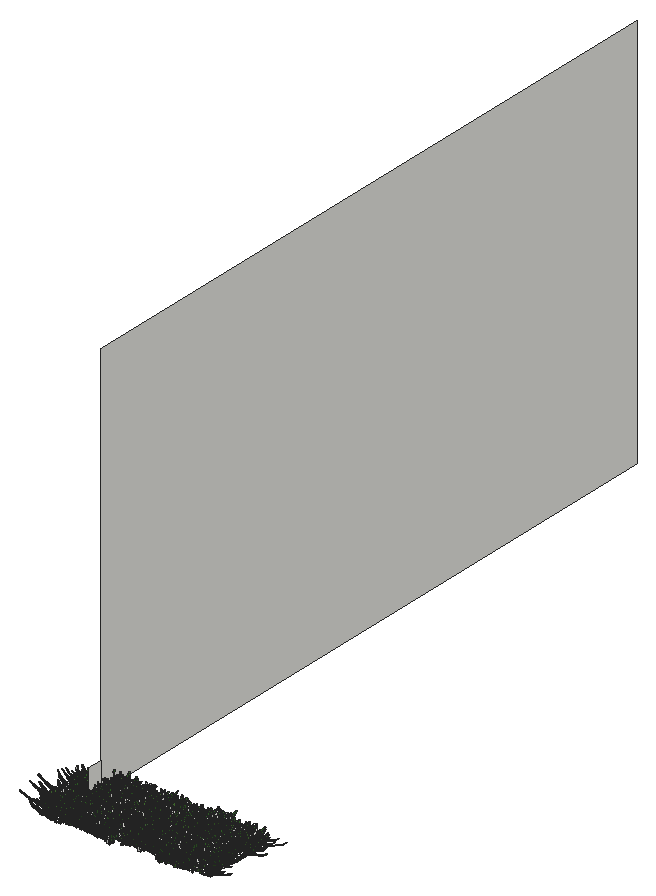
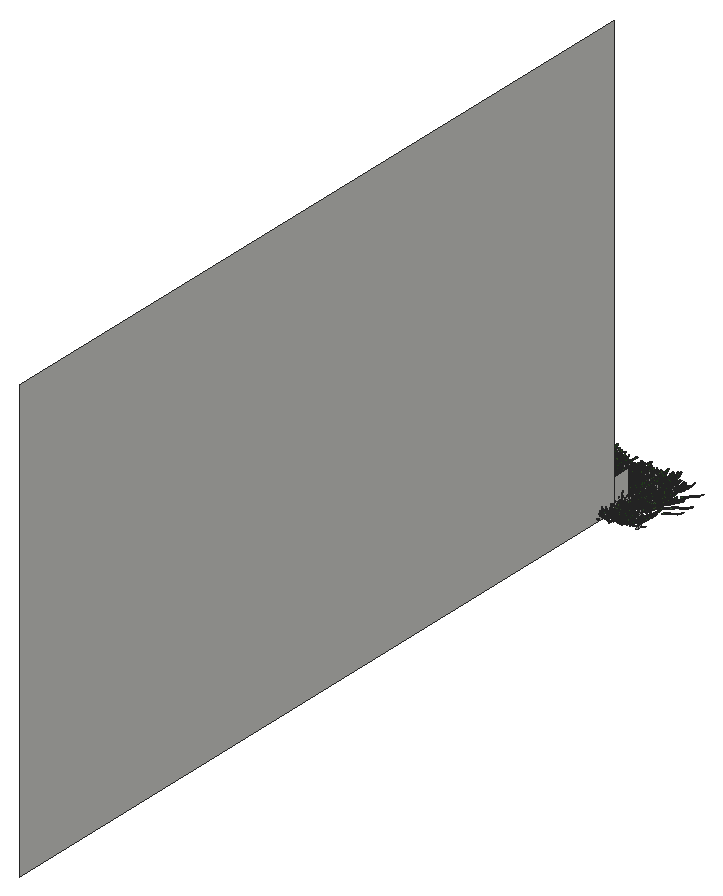
# SketchUp Ruby script. Lengths in inches.
U = 1.inch
M = Sketchup.active_model
def pt(a) = Geom::Point3d.new(a.map { |v| v * U })
def face(e, loops, mat)
  f = e.add_face(loops[0].map { |a| pt(a) })
  loops[1..].each { |l| e.add_face(l.map { |a| pt(a) }).erase! }
  f.material = f.back_material = mat if mat
  f
end
# faces: each face lists its corners as indices into pts; further lists are holes
def faces(e, pts, list, mat = nil) = list.each { |f| face(e, (f[0].is_a?(Array) ? f : [f]).map { |l| l.map { |i| pts[i] } }, mat) }
# xy, xz, yz: faces in a plane at the given z, y or x. An outline is a flat list of corners, or four numbers for a rectangle; further outlines are holes
def ring(l) = l.size == 4 ? [[l[0], l[1]], [l[2], l[1]], [l[2], l[3]], [l[0], l[3]]] : l.each_slice(2).to_a
def flat(e, list, mat, &to3) = list.each { |f| face(e, (f[0].is_a?(Array) ? f : [f]).map { |l| ring(l).map { |u, v| to3.(u, v) } }, mat) }
def xy(e, z, list, mat = nil) = flat(e, list, mat) { |x, y| [x, y, z] }
def xz(e, y, list, mat = nil) = flat(e, list, mat) { |x, z| [x, y, z] }
def yz(e, x, list, mat = nil) = flat(e, list, mat) { |y, z| [x, y, z] }
def lines(e, pts, list) = list.each { |a, b| e.add_line(pt(pts[a]), pt(pts[b])) }
# prism: a flat outline (further loops are holes) pulled along v
def prism(e, loops, v, mat = nil)
  f = face(e, loops, mat); d = Geom::Vector3d.new(v.map { |x| x * U })
  f.pushpull(f.normal.samedirection?(d) ? d.length : -d.length)
end
def box(e, o, s, mat = nil) = prism(e, [[o, [o[0] + s[0], o[1], o[2]], [o[0] + s[0], o[1] + s[1], o[2]], [o[0], o[1] + s[1], o[2]]]], [0, 0, s[2]], mat)
def at(x, y, z, deg = 0) = Geom::Transformation.translation(pt([x, y, z])) * Geom::Transformation.rotation(ORIGIN, Z_AXIS, deg.degrees)
def axes(o, x, y, z) = Geom::Transformation.new([*x, 0, *y, 0, *z, 0, *pt(o).to_a, 1])
def part(name) = M.definitions.add(name)
# library, detail: a bought-in or finely detailed component or shape, given as its bounding box
def library(name, o, s) = part(name).tap { |d| box(d.entities, o, s) }
def detail(e, o, s) = box(e.add_group.entities, o, s)
def put(e, d, t, mat = nil) = e.add_instance(d, t).tap { |i| i.material = mat if mat }
def group(e, t, mat = nil) = e.add_group.tap { |g| g.transformation = t; g.material = mat if mat }.entities
root = M.entities
M.materials.add("Material82").color = [68, 110, 58]
M.materials.add("Material83").color = [48, 90, 38]
M.materials.add("Material84").color = [68, 110, 48]
M.materials.add("Material85").color = [48, 90, 48]
M.materials.add("Material86").color = [58, 110, 58]
M.materials.add("Material87").color = [58, 90, 38]
M.materials.add("Material88").color = [68, 100, 58]
M.materials.add("Material89").color = [48, 100, 38]
c1 = part("grass00")
p = [[-0.6875,0.15,0],[-0.56,0.08,5.52],[-0.04,0.03,2.76],[0.48,-0.02,0],[0.35,-0.02,5.52],[-0.1,-0.14,5.52],
  [-0.12,0.65,8.37],[-0.42,0.65,8.37]]
faces(c1.entities,p,[[0,1,2,3],[3,2,4],[1,5,2],[5,4,2],[1,6,5],[4,5,6],[7,6,1]])
c2 = part("Group16\#1")
put(c2.entities,c1,axes([1.44,-0.61,-0.01],[0.05352,0.12609,0],[-0.10704,0.04543,0.07239],[0.06664,-0.02828,0.11628]),"Material85")
put(c2.entities,c1,axes([0.76,-0.15,-0.01],[0.04676,0.24062,0],[-0.23162,0.04501,0.06642],[0.0652,-0.01267,0.23595]),"Material82")
put(c2.entities,c1,axes([0.79,0.01,-0.01],[-0.00606,0.34651,0],[-0.34381,-0.00602,0.0432],[0.04319,0.00076,0.34386]))
put(c2.entities,c1,axes([1,0.23,-0.01],[-0.07192,0.31144,0],[-0.28722,-0.06632,0.1236],[0.12043,0.02781,0.29478]),"Material84")
put(c2.entities,c1,axes([1.66,0.77,-0.01],[-0.13828,0.29651,0],[-0.21551,-0.1005,0.22471],[0.20365,0.09498,0.23779]),"Material89")
put(c2.entities,c1,axes([0.6875,0.52,-0.01],[-0.18126,0.24051,0],[-0.22746,-0.17142,0.09788],[0.07817,0.05891,0.28481]),"Material84")
put(c2.entities,c1,axes([0.68,0.78,-0.01],[-0.215,0.18688,0],[-0.12385,-0.14248,0.21334],[0.13995,0.16101,0.18878]),"Material82")
put(c2.entities,c1,axes([0.56,1,-0.01],[-0.13756,0.07624,0],[-0.06159,-0.11112,0.0927],[0.04494,0.08108,0.12705]),"Material84")
put(c2.entities,c1,axes([0.2,0.64,-0.01],[-0.23729,0.07254,0],[-0.05711,-0.18681,0.153],[0.04473,0.14632,0.19535]),"Material89")
put(c2.entities,c1,axes([0.0625,0.72,-0.01],[-0.28874,0.02525,0],[-0.02179,-0.24916,0.14647],[0.01276,0.14591,0.25012]),"Material82")
put(c2.entities,c1,axes([-0.08,0.62,-0.01],[-0.34089,-0.04187,0],[0.03255,-0.26504,0.216],[-0.02633,0.21439,0.26703]),"Material89")
put(c2.entities,c1,axes([-0.34,0.98,-0.01],[-0.14314,-0.0493,0],[0.04397,-0.12769,0.06843],[-0.02228,0.0647,0.13505]),"Material89")
put(c2.entities,c1,axes([-0.87,1.45,-0.01],[-0.23488,-0.14114,0],[0.13761,-0.22901,0.06087],[-0.03135,0.05217,0.26717]))
put(c2.entities,c1,axes([-0.72,0.77,-0.01],[-0.14208,-0.13251,0],[0.07209,-0.0773,0.16301],[-0.11118,0.11922,0.1057]),"Material89")
put(c2.entities,c1,axes([-0.62,0.43,-0.01],[-0.14845,-0.21203,0],[0.18654,-0.13061,0.12304],[-0.10079,0.07057,0.22772]),"Material82")
put(c2.entities,c1,axes([-0.68,0.29,-0.01],[-0.13639,-0.32136,0],[0.31723,-0.13464,0.05579],[-0.05136,0.0218,0.34462]),"Material83")
put(c2.entities,c1,axes([-0.64,0.125,-0.01],[-0.0458,-0.23569,0],[0.22124,-0.043,0.08276],[-0.08124,0.01579,0.22538]),"Material86")
put(c2.entities,c1,axes([-1.6,-0.03,-0.01],[0.00576,-0.32897,0],[0.27526,0.00482,0.18018],[-0.18015,-0.00315,0.2753]),"Material84")
put(c2.entities,c1,axes([-1.36,-0.31,-0.01],[0.05718,-0.24765,0],[0.18172,0.04196,0.17267],[-0.16825,-0.03885,0.1865]),"Material89")
put(c2.entities,c1,axes([-1.54,-0.72,-0.01],[0.06537,-0.14017,0],[0.13555,0.06321,0.03939],[-0.0357,-0.01665,0.14956]))
put(c2.entities,c1,axes([-1.19,-0.9,-0.01],[0.09597,-0.12735,0],[0.11214,0.08451,0.07557],[-0.06035,-0.04548,0.14042]),"Material88")
put(c2.entities,c1,axes([-0.47,-0.54,-0.01],[0.11588,-0.10072,0],[0.0618,0.0711,0.12124],[-0.07953,-0.0915,0.0942]))
put(c2.entities,c1,axes([-0.47,-0.84,-0.01],[0.11927,-0.0661,0],[0.06603,0.11913,0.00646],[-0.00313,-0.00565,0.13621]),"Material84")
put(c2.entities,c1,axes([-0.38,-1.24,-0.01],[0.28037,-0.08571,0],[0.0618,0.20215,0.20315],[-0.05939,-0.19428,0.21139]),"Material88")
put(c2.entities,c1,axes([-0.06,-0.66,-0.01],[0.22719,-0.01987,0],[0.01247,0.14255,0.17758],[-0.01547,-0.17691,0.1431]),"Material87")
put(c2.entities,c1,axes([0.11,-0.89,-0.01],[0.14882,0.01828,0],[-0.01058,0.08611,0.12229],[0.01491,-0.12138,0.08676]),"Material85")
put(c2.entities,c1,axes([0.25,-0.72,-0.01],[0.20481,0.07053,0],[-0.06206,0.18022,0.10291],[0.03351,-0.0973,0.1906]),"Material85")
put(c2.entities,c1,axes([0.85,-1.42,-0.01],[0.16481,0.09904,0],[-0.09472,0.15762,0.05616],[0.02893,-0.04814,0.18389]),"Material84")
put(c2.entities,c1,axes([1.01,-1.09,-0.01],[0.21858,0.20385,0],[-0.17495,0.1876,0.15339],[0.10462,-0.11218,0.25652]),"Material89")
put(c2.entities,c1,axes([1.01,-0.71,-0.01],[0.08733,0.12473,0],[-0.06445,0.04512,0.13037],[0.1068,-0.07477,0.07867]),"Material85")
c3 = part("Group15\#1")
put(c3.entities,c2,at(0,0,0))
c4 = part("3darcstudiotree_grass00\#1")
put(c4.entities,c3,at(0,0,0))
yz(root,782.4375,[[1040.81,-29.74,1046.93,-18.36],[1046.93,-29.74,1318.18,131.1875]])
put(root,c4,axes([780.74,1025.45,-29.74],[3.43874,0.27286,0],[-0.6732,1.31953,-0.0192],[-0.02432,0.04768,1.64321]))
put(root,c4,axes([802.54,1025.03,-29.74],[-4.04807,0.23611,0],[-0.60438,-1.61163,-0.04443],[-0.03837,-0.10233,1.82802]))
put(root,c4,axes([782.67,1025.28,-29.74],[1.27855,1.29921,0],[-4.02019,0.61532,-0.04732],[-0.19364,0.02964,1.41896]))
put(root,c4,axes([828.62,1025.53,-29.74],[-1.72673,1.11938,0],[-3.66172,-0.8785,-0.02284],[-0.09991,-0.02397,1.64481]))
put(root,c4,axes([791.75,1026.65,-29.74],[1.05791,1.29898,0],[-3.4169,0.4328,-0.04361],[-0.24845,0.03147,1.60948]))
put(root,c4,axes([834.85,1027.24,-29.74],[2.97779,-1.31333,0],[2.93322,1.03437,-0.03435],[0.15944,0.05623,1.83666]))
put(root,c4,axes([804.76,1027.35,-29.74],[1.68348,-1.42,0],[3.90393,0.71983,-0.01397],[0.0682,0.01258,1.74087]))
put(root,c4,axes([786.06,1027.47,-29.74],[-2.53432,-1.16731,0],[3.13366,-1.05813,-0.03189],[0.12006,-0.04054,1.53238]))
put(root,c4,axes([795.22,1027.46,-29.74],[-1.68076,1.66641,0],[-3.14491,-0.49334,-0.04072],[-0.22908,-0.03594,1.53595]))
put(root,c4,axes([821.7,1027.81,-29.74],[-3.64575,-0.40954,0],[1.09452,-1.51542,-0.03955],[0.07063,-0.09779,1.95202]))
put(root,c4,axes([812.24,1027.78,-29.74],[-4.50339,0.12702,0],[-0.32923,-1.8154,-0.06114],[-0.02191,-0.12082,1.73764]))
put(root,c4,axes([826.89,1028.21,-29.74],[3.9368,0.32867,0],[-0.7645,1.42421,-0.03259],[-0.03941,0.07343,1.61556]))
put(root,c4,axes([799.375,1028.19,-29.74],[-1.97756,-1.20873,0],[2.87461,-0.73146,-0.04434],[0.19177,-0.0488,1.31982]))
put(root,c4,axes([838.74,1027.84,-29.74],[-0.96856,1.32293,0],[-4.17213,-0.47507,-0.01983],[-0.0846,-0.00963,1.44555]))
put(root,c4,axes([816.35,1028.02,-29.74],[-4.11343,-0.37841,0],[0.77008,-1.30194,-0.01564],[0.01915,-0.03238,1.3694]))
put(root,c4,axes([791.55,1029.24,-29.74],[3.30112,0.44872,0],[-1.07202,1.22659,-0.01199],[-0.02088,0.02389,1.31812]))
put(root,c4,axes([782.47,1029.07,-29.74],[2.54447,1.0037,0],[-2.66541,1.05092,-0.04694],[-0.19938,0.07861,1.69685]))
put(root,c4,axes([795.87,1029.17,-29.74],[1.71949,1.25443,0],[-3.5766,0.76249,-0.00296],[-0.01327,0.00283,1.55057]))
put(root,c4,axes([828.32,1028.93,-29.74],[-0.85979,1.68043,0],[-3.51636,-0.27982,-0.00527],[-0.03686,-0.00293,1.91768]))
put(root,c4,axes([802.46,1030.125,-29.74],[2.98286,-1.36319,0],[2.94856,1.00345,-0.04774],[0.23651,0.08049,1.91023]))
put(root,c4,axes([780.62,1029.47,-29.74],[-4.5512,0.12899,0],[-0.29843,-1.6376,-0.01837],[-0.00647,-0.03552,1.53349]))
put(root,c4,axes([833.1,1030.28,-29.74],[2.31859,-1.24057,0],[3.7429,1.08799,-0.00987],[0.04342,0.01262,1.9048]))
put(root,c4,axes([806.14,1029.86,-29.74],[3.00883,1.26771,0],[-3.0504,1.12602,-0.05678],[-0.17699,0.06533,1.337]))
put(root,c4,axes([818.37,1030.28,-29.74],[2.02967,-1.41693,0],[3.62772,0.8082,-0.05349],[0.29346,0.06538,1.96798]))
put(root,c4,axes([823.69,1030.18,-29.74],[-1.26608,-1.23533,0],[3.94424,-0.62872,-0.05241],[0.25484,-0.04062,1.67241]))
put(root,c4,axes([811.92,1030.22,-29.74],[-2.51394,1.47726,0],[-3.35133,-0.88701,-0.03945],[-0.17377,-0.04599,1.6047]))
put(root,c4,axes([782.69,1031.4375,-29.74],[1.0408,-1.70786,0],[3.59221,0.34047,-0.00397],[0.02558,0.00242,1.83602]))
put(root,c4,axes([835.27,1031.08,-29.74],[1.31466,1.33352,0],[-4.27103,0.65487,-0.01993],[-0.10773,0.01652,1.99239]))
put(root,c4,axes([829.86,1031.4,-29.74],[3.99583,0.96728,0],[-1.88023,1.20803,-0.0354],[-0.13352,0.08578,1.94218]))
put(root,c4,axes([801.69,1031.29,-29.74],[1.07934,1.49635,0],[-4.41478,0.49528,-0.01266],[-0.0607,0.00681,1.71446]))
put(root,c4,axes([790.3,1031.48,-29.74],[-3.99444,-0.7583,0],[1.47781,-1.21073,-0.01121],[0.03612,-0.02959,1.89718]))
put(root,c4,axes([822.25,1031.38,-29.74],[0.15484,1.66312,0],[-4.06716,0.05889,-0.05084],[-0.28361,0.00411,1.70302]))
put(root,c4,axes([807.62,1031.78,-29.74],[1.72171,1.1824,0],[-3.73214,0.84521,-0.0451],[-0.23455,0.05312,1.93445]))
put(root,c4,axes([818.36,1032.42,-29.74],[0.19619,-1.71635,0],[3.31321,0.0589,-0.03915],[0.30696,0.00546,1.95085]))
put(root,c4,axes([795.96,1032.2,-29.74],[-0.66988,1.5554,0],[-4.19746,-0.28116,-0.06003],[-0.34231,-0.02293,1.84592]))
put(root,c4,axes([779.55,1032.45,-29.74],[-1.94069,1.13311,0],[-3.87728,-1.03282,-0.01862],[-0.08293,-0.02209,1.88514]))
put(root,c4,axes([807.42,1033.21,-29.74],[1.1935,-1.34336,0],[4.3339,0.59885,-0.02001],[0.09738,0.01346,1.77455]))
put(root,c4,axes([811.17,1032.45,-29.74],[-2.50228,1.03927,0],[-3.36492,-1.26006,-0.01749],[-0.0653,-0.02445,1.7911]))
put(root,c4,axes([821.2,1033.83,-29.74],[3.2454,-0.59836,0],[1.90263,1.60498,-0.04906],[0.1129,0.09524,1.82977]))
put(root,c4,axes([802.49,1034.125,-29.74],[3.36205,-0.0702,0],[0.18049,1.34442,-0.02933],[0.01197,0.08919,1.97542]))
put(root,c4,axes([838.15,1033.98,-29.74],[-3.24576,-0.77305,0],[1.70346,-1.11239,-0.04514],[0.15554,-0.10157,1.64638]))
put(root,c4,axes([810.92,1033.62,-29.74],[-2.83529,0.94791,0],[-2.49489,-1.16063,-0.0209],[-0.0692,-0.03219,1.48072]))
put(root,c4,axes([817.75,1033.95,-29.74],[-4.36996,-0.43983,0],[0.81337,-1.25688,-0.00096],[0.00152,-0.00235,1.58162]))
put(root,c4,axes([782.19,1034.09,-29.74],[2.0306,1.51402,0],[-3.86929,0.80712,-0.01033],[-0.04249,0.00886,1.52631]))
put(root,c4,axes([791.42,1034.66,-29.74],[4.32541,0.68003,0],[-1.26335,1.24977,-0.02018],[-0.04043,0.04,1.38364]))
put(root,c4,axes([828.54,1034.46,-29.74],[-1.11192,1.29739,0],[-3.39488,-0.45252,-0.04196],[-0.24016,-0.03201,1.62262]))
put(root,c4,axes([796.08,1034.66,-29.74],[-3.14118,-0.50543,0],[1.51948,-1.46871,-0.03312],[0.08056,-0.07787,1.94116]))
put(root,c4,axes([835.37,1034.5,-29.74],[-3.94382,0.34286,0],[-0.79478,-1.42188,-0.01188],[-0.01845,-0.03301,1.99665]))
put(root,c4,axes([780.03,1034.6,-29.74],[-4.08544,0.78173,0],[-2.02978,-1.64985,-0.06144],[-0.10479,-0.08517,1.3618]))
put(root,c4,axes([817.55,1035.39,-29.74],[0.47621,-1.80202,0],[3.38439,0.1391,-0.02929],[0.17813,0.00732,1.55926]))
put(root,c4,axes([832.73,1035.93,-29.74],[4.51376,-0.38644,0],[0.93116,1.69158,-0.03342],[0.04124,0.07493,1.91382]))
put(root,c4,axes([800.54,1036.43,-29.74],[2.93855,-0.93601,0],[2.3882,1.16609,-0.03491],[0.14245,0.06955,1.84986]))
put(root,c4,axes([788.35,1036.26,-29.74],[3.70843,0.7821,0],[-1.67561,1.2357,-0.00407],[-0.01146,0.00845,1.59208]))
put(root,c4,axes([810.48,1036.17,-29.74],[-3.51736,-0.62046,0],[1.43276,-1.26324,-0.00732],[0.0191,-0.01684,1.68082]))
put(root,c4,axes([826.86,1036.67,-29.74],[1.17526,-1.64902,0],[4.03097,0.44682,-0.04021],[0.21409,0.02373,1.73573]))
put(root,c4,axes([824.59,1036.78,-29.74],[3.33693,-0.09981,0],[0.31842,1.6558,-0.06006],[0.02203,0.11454,1.53056]))
put(root,c4,axes([795.02,1036.95,-29.74],[1.17971,-1.62892,0],[3.63954,0.40996,-0.01145],[0.05532,0.00623,1.42532]))
put(root,c4,axes([805.33,1036.61,-29.74],[-2.4369,-0.91248,0],[2.76412,-1.14811,-0.01822],[0.07791,-0.03236,1.86907]))
put(root,c4,axes([783.25,1036.76,-29.74],[-4.28311,0.42951,0],[-0.86146,-1.33607,-0.01716],[-0.03026,-0.04692,1.87475]))
put(root,c4,axes([785.52,1037.51,-29.74],[3.93391,0.38635,0],[-0.92741,1.4687,-0.04825],[-0.05916,0.09369,1.45973]))
put(root,c4,axes([797.27,1037.91,-29.74],[1.5424,-1.39232,0],[4.02917,0.6942,-0.02716],[0.11079,0.01909,1.46706]))
put(root,c4,axes([805.98,1037.73,-29.74],[-3.14575,-1.33265,0],[2.56413,-0.94137,-0.04944],[0.22162,-0.08136,1.60821]))
put(root,c4,axes([822.71,1037.98,-29.74],[3.16271,-0.89527,0],[1.91794,1.05379,-0.02763],[0.08663,0.0476,1.3256]))
put(root,c4,axes([788.07,1037.89,-29.74],[2.84603,0.80034,0],[-2.3016,1.27293,-0.03635],[-0.10022,0.05543,1.41103]))
put(root,c4,axes([813.56,1037.97,-29.74],[2.37182,1.09167,0],[-3.5393,1.19596,-0.05975],[-0.18065,0.06104,1.3909]))
put(root,c4,axes([817.36,1038.71,-29.74],[1.48234,-1.44208,0],[4.35208,0.69577,-0.03495],[0.16928,0.02706,1.83937]))
put(root,c4,axes([779.16,1038,-29.74],[-3.86986,1.0079,0],[-2.20275,-1.31539,-0.01955],[-0.05283,-0.03155,1.46911]))
put(root,c4,axes([832.99,1038.87,-29.74],[2.23867,-1.3669,0],[3.69886,0.94218,-0.0579],[0.27243,0.06939,1.84885]))
put(root,c4,axes([829.05,1038.61,-29.74],[-1.90503,-1.23869,0],[3.27066,-0.78232,-0.01057],[0.0584,-0.01397,1.85267]))
put(root,c4,axes([799.68,1038.94,-29.74],[-2.84152,0.97731,0],[-2.62045,-1.18497,-0.0546],[-0.22213,-0.10045,1.84968]))
put(root,c4,axes([797.36,1039.74,-29.74],[-2.28475,-0.97473,0],[2.77585,-1.01196,-0.01026],[0.04604,-0.01678,1.73127]))
put(root,c4,axes([826.72,1039.7,-29.74],[1.07114,1.64692,0],[-4.05863,0.41055,-0.04684],[-0.20509,0.02075,1.41954]))
put(root,c4,axes([791.17,1039.79,-29.74],[0.72726,1.40914,0],[-3.71927,0.29854,-0.02796],[-0.18755,0.01505,1.94708]))
put(root,c4,axes([807.54,1040.33,-29.74],[-2.0126,-1.62184,0],[4.11765,-0.79471,-0.06506],[0.29073,-0.05611,1.70958]))
put(root,c4,axes([799.85,1039.74,-29.74],[-3.10197,1.07124,0],[-2.38472,-1.07399,-0.00238],[-0.01101,-0.00496,1.90825]))
put(root,c4,axes([817.04,1039.99,-29.74],[-3.67787,-0.26396,0],[0.66039,-1.43112,-0.02729],[0.03307,-0.07167,1.8715]))
put(root,c4,axes([824.17,1040.55,-29.74],[-0.88129,-1.68738,0],[3.67182,-0.29826,-0.02826],[0.15697,-0.01275,1.59374]))
put(root,c4,axes([784.72,1040.8125,-29.74],[-1.15236,-1.67434,0],[3.65122,-0.39084,-0.0298],[0.14551,-0.01558,1.43464]))
put(root,c4,axes([834.2,1040.57,-29.74],[0.85919,1.59494,0],[-3.67668,0.30804,-0.01067],[-0.0678,0.00568,1.82972]))
put(root,c4,axes([810.89,1041.01,-29.74],[0.845,1.5364,0],[-3.22221,0.27563,-0.00976],[-0.06274,0.00537,1.62508]))
put(root,c4,axes([835.375,1042.06,-29.74],[3.21747,0.34612,0],[-1.00705,1.45598,-0.00322],[-0.00588,0.0085,1.99197]))
put(root,c4,axes([807.11,1042.35,-29.74],[2.05313,-1.14667,0],[3.04328,0.84748,-0.00946],[0.04471,0.01245,1.61646]))
put(root,c4,axes([827.93,1042.28,-29.74],[-2.06721,-1.47479,0],[2.97534,-0.64864,-0.04183],[0.21369,-0.04658,1.48723]))
put(root,c4,axes([813.83,1042.34,-29.74],[3.55632,0.05998,0],[-0.17821,1.64336,-0.05798],[-0.01271,0.11725,1.60438]))
put(root,c4,axes([838.15,1042,-29.74],[-3.26011,-0.21751,0],[0.57833,-1.34815,-0.02254],[0.02017,-0.04702,1.39425]))
put(root,c4,axes([795.2,1043.2,-29.74],[3.71353,-0.51552,0],[1.56304,1.75115,-0.03514],[0.05159,0.0578,1.55988]))
put(root,c4,axes([816.91,1043.27,-29.74],[1.06558,-1.7102,0],[3.88793,0.37676,-0.05295],[0.33853,0.03281,1.97565]))
put(root,c4,axes([778.73,1043.27,-29.74],[3.5779,0.22372,0],[-0.65952,1.64048,-0.02805],[-0.02776,0.06904,1.99488]))
put(root,c4,axes([789.66,1043.23,-29.74],[-0.99859,-1.42329,0],[3.17499,-0.34645,-0.0133],[0.07574,-0.00827,1.45899]))
put(root,c4,axes([784.95,1042.7,-29.74],[-2.82382,0.83563,0],[-2.68315,-1.4102,-0.02868],[-0.0714,-0.03753,1.39]))
put(root,c4,axes([823.84,1043.07,-29.74],[-4.01729,-0.17274,0],[0.40562,-1.46709,-0.05296],[0.03317,-0.11998,1.62079]))
put(root,c4,axes([800.72,1043.13,-29.74],[-1.96777,1.0795,0],[-3.29786,-0.93497,-0.0015],[-0.00541,-0.00153,1.35234]))
put(root,c4,axes([818.03,1044.2,-29.74],[3.84561,-0.02617,0],[0.07345,1.67847,-0.0287],[0.00308,0.07036,1.98369]))
put(root,c4,axes([794.53,1044.41,-29.74],[1.96372,-1.5045,0],[4.10696,0.83372,-0.06088],[0.26019,0.05282,1.6642]))
put(root,c4,axes([807.39,1044.37,-29.74],[3.54187,-0.26159,0],[0.80325,1.69151,-0.05648],[0.04449,0.09368,1.39957]))
put(root,c4,axes([789.46,1044.66,-29.74],[1.82247,1.66574,0],[-4.14446,0.70523,-0.02206],[-0.09849,0.01676,1.64521]))
put(root,c4,axes([813.33,1044.38,-29.74],[-3.99369,0.93834,0],[-2.11578,-1.40055,-0.00882],[-0.02078,-0.01375,1.42641]))
put(root,c4,axes([827.21,1044.57,-29.74],[-3.34892,0.63546,0],[-1.79553,-1.4717,-0.05656],[-0.12201,-0.10001,1.54444]))
put(root,c4,axes([823.42,1044.64,-29.74],[-2.29973,1.37871,0],[-3.78776,-0.98265,-0.04701],[-0.18775,-0.04871,1.62457]))
put(root,c4,axes([837.6,1045.39,-29.74],[4.21864,0.55626,0],[-1.1609,1.36932,-0.01696],[-0.03551,0.04188,1.81122]))
put(root,c4,axes([801.27,1044.99,-29.74],[-0.80631,1.56039,0],[-4.1673,-0.33492,-0.00834],[-0.04436,-0.00356,1.72954]))
put(root,c4,axes([833.45,1045.37,-29.74],[-3.37719,0.09425,0],[-0.3007,-1.67585,-0.01026],[-0.00386,-0.0215,1.70108]))
put(root,c4,axes([785.75,1045.54,-29.74],[-1.94441,1.40342,0],[-3.94861,-0.85085,-0.04785],[-0.22127,-0.04768,1.77706]))
put(root,c4,axes([834.36,1046.53,-29.74],[3.52188,-1.04915,0],[2.07703,1.0844,-0.01203],[0.05383,0.0281,1.91781]))
put(root,c4,axes([812.14,1046.875,-29.74],[1.01558,-1.39222,0],[4.1939,0.47581,-0.0144],[0.07646,0.00867,1.80693]))
put(root,c4,axes([799.58,1046.35,-29.74],[0.28845,1.63387,0],[-3.6901,0.10132,-0.01352],[-0.07291,0.002,1.49862]))
put(root,c4,axes([782.34,1047.07,-29.74],[1.87129,-1.65871,0],[3.35394,0.58849,-0.03607],[0.16948,0.02974,1.41495]))
put(root,c4,axes([838.03,1047.05,-29.74],[3.01548,-1.43579,0],[2.66285,0.86981,-0.04892],[0.23141,0.07559,1.59182]))
put(root,c4,axes([829.35,1046.41,-29.74],[-3.21998,0.77713,0],[-2.13854,-1.37813,-0.04749],[-0.1058,-0.06818,1.3106]))
put(root,c4,axes([821.78,1047.21,-29.74],[4.18213,-0.23196,0],[0.63555,1.78214,-0.01318],[0.01066,0.02989,1.98636]))
put(root,c4,axes([794.35,1047.34,-29.74],[4.18444,0.27637,0],[-0.72897,1.71663,-0.00046],[-0.00033,0.00077,1.40239]))
put(root,c4,axes([806.84,1047.39,-29.74],[3.48402,0.19943,0],[-0.6366,1.72969,-0.0224],[-0.01372,0.03729,1.41716]))
put(root,c4,axes([791.57,1047.47,-29.74],[2.76674,0.9412,0],[-2.67302,1.22208,-0.02494],[-0.08686,0.03971,1.63549]))
put(root,c4,axes([818.46,1047.78,-29.74],[1.32588,-1.61709,0],[3.49004,0.44505,-0.02554],[0.12415,0.01583,1.40467]))
put(root,c4,axes([779.52,1047.58,-29.74],[3.90165,0.71674,0],[-1.5443,1.30747,-0.0112],[-0.02712,0.02296,1.5714]))
put(root,c4,axes([791.08,1048.63,-29.74],[2.92757,-1.05075,0],[2.58194,1.11883,-0.00947],[0.03015,0.01306,1.36019]))
put(root,c4,axes([813.3,1048.73,-29.74],[2.43403,-1.47369,0],[3.95187,1.01516,-0.04483],[0.17665,0.04538,1.66248]))
put(root,c4,axes([799.73,1048.72,-29.74],[-0.61871,-1.33799,0],[4.52735,-0.32561,-0.01194],[0.05418,-0.0039,1.59034]))
put(root,c4,axes([824.47,1048.99,-29.74],[-2.58829,-1.32174,0],[3.13096,-0.95358,-0.00917],[0.03927,-0.01196,1.60374]))
put(root,c4,axes([835.99,1048.77,-29.74],[0.77928,1.7442,0],[-4.29167,0.29822,-0.04576],[-0.22745,0.0158,1.64855]))
put(root,c4,axes([806.36,1048.96,-29.74],[-0.96871,1.48497,0],[-4.54289,-0.46091,-0.03008],[-0.14643,-0.01486,1.76703]))
put(root,c4,axes([777.25,1049.47,-29.74],[2.90547,0.96842,0],[-2.50521,1.16898,-0.00305],[-0.01073,0.00501,1.58836]))
put(root,c4,axes([795.18,1049.27,-29.74],[-3.42471,-0.0278,0],[0.09598,-1.83904,-0.05231],[0.00587,-0.11256,1.90792]))
put(root,c4,axes([784.54,1049.57,-29.74],[-1.92512,-1.14787,0],[3.14134,-0.81939,-0.00554],[0.02611,-0.00681,1.59445]))
put(root,c4,axes([826.88,1049.59,-29.74],[2.80131,1.49669,0],[-2.81369,0.81906,-0.03251],[-0.16371,0.04766,1.64081]))
put(root,c4,axes([817.75,1050.04,-29.74],[-2.36734,0.93793,0],[-2.35302,-0.92369,-0.04592],[-0.18701,-0.07341,1.42994]))
put(root,c4,axes([801.67,1050.73,-29.74],[-4.54557,-0.49368,0],[1.16722,-1.67149,-0.00177],[0.00248,-0.00355,1.73275]))
put(root,c4,axes([817.37,1051.27,-29.74],[2.58784,1.12355,0],[-2.76399,0.99014,-0.01914],[-0.07187,0.02574,1.41957]))
put(root,c4,axes([832.34,1051.83,-29.74],[3.2252,-1.24507,0],[3.05222,1.22967,-0.00616],[0.02183,0.0088,1.65812]))
put(root,c4,axes([790.77,1051.09,-29.74],[-3.2702,-0.26148,0],[0.88726,-1.72581,-0.02938],[0.02304,-0.04482,1.3208]))
put(root,c4,axes([785.25,1051.72,-29.74],[3.46613,-0.34597,0],[1.04996,1.63602,-0.03471],[0.05136,0.08002,1.93398]))
put(root,c4,axes([838.6875,1051.19,-29.74],[-1.83571,1.27258,0],[-3.25848,-0.73105,-0.04597],[-0.18825,-0.04223,1.32398]))
put(root,c4,axes([824.41,1051.87,-29.74],[3.30404,-0.44467,0],[1.11823,1.29225,-0.02189],[0.05068,0.05857,1.86062]))
put(root,c4,axes([809.98,1051.79,-29.74],[3.79709,-0.21086,0],[0.51761,1.44966,-0.04526],[0.04066,0.11387,1.7925]))
put(root,c4,axes([805.09,1051.42,-29.74],[-1.13728,1.56272,0],[-3.25789,-0.36875,-0.04255],[-0.28342,-0.03208,1.76068]))
put(root,c4,axes([793.87,1052.16,-29.74],[3.34396,-0.78628,0],[2.01461,1.33256,-0.01626],[0.05098,0.03372,1.80561]))
put(root,c4,axes([827.4,1051.57,-29.74],[-3.32221,0.63503,0],[-1.46009,-1.18802,-0.04774],[-0.13797,-0.11226,1.66266]))
put(root,c4,axes([789.58,1052.89,-29.74],[1.37568,-1.20584,0],[3.91752,0.6951,-0.04402],[0.22671,0.04023,1.81837]))
put(root,c4,axes([811.8,1052.8,-29.74],[3.59871,0.46514,0],[-1.32691,1.59666,-0.04711],[-0.07156,0.0861,1.55738]))
put(root,c4,axes([799.57,1053,-29.74],[-2.0544,-1.27697,0],[2.98947,-0.74801,-0.00968],[0.05342,-0.01337,1.73508]))
put(root,c4,axes([838.51,1053.42,-29.74],[3.62221,-0.68496,0],[1.51778,1.24833,-0.03326],[0.08982,0.07387,1.64345]))
put(root,c4,axes([829.74,1052.98,-29.74],[-0.69326,1.7064,0],[-4.31448,-0.27262,-0.01053],[-0.04979,-0.00315,1.56894]))
put(root,c4,axes([825.05,1053.3125,-29.74],[2.26243,1.54744,0],[-3.43917,0.78203,-0.02249],[-0.10645,0.02421,1.62577]))
